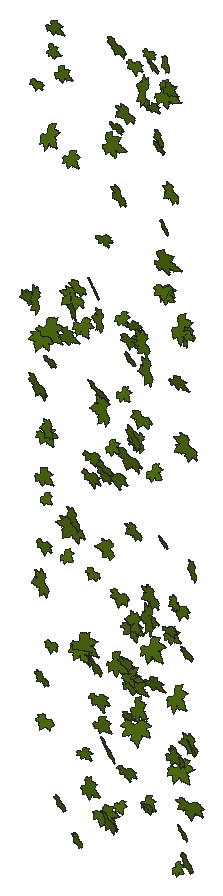
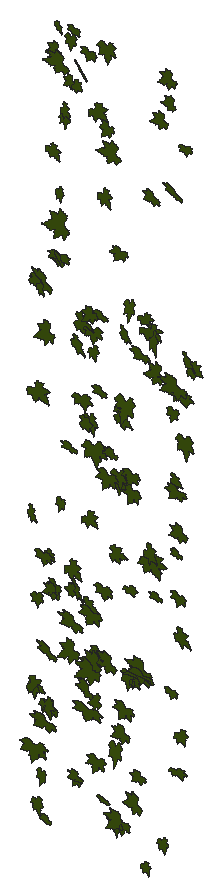
# SketchUp Ruby script. Lengths in inches.
U = 1.inch
M = Sketchup.active_model
def pt(a) = Geom::Point3d.new(a.map { |v| v * U })
def face(e, loops, mat)
  f = e.add_face(loops[0].map { |a| pt(a) })
  loops[1..].each { |l| e.add_face(l.map { |a| pt(a) }).erase! }
  f.material = f.back_material = mat if mat
  f
end
# faces: each face lists its corners as indices into pts; further lists are holes
def faces(e, pts, list, mat = nil) = list.each { |f| face(e, (f[0].is_a?(Array) ? f : [f]).map { |l| l.map { |i| pts[i] } }, mat) }
# xy, xz, yz: faces in a plane at the given z, y or x. An outline is a flat list of corners, or four numbers for a rectangle; further outlines are holes
def ring(l) = l.size == 4 ? [[l[0], l[1]], [l[2], l[1]], [l[2], l[3]], [l[0], l[3]]] : l.each_slice(2).to_a
def flat(e, list, mat, &to3) = list.each { |f| face(e, (f[0].is_a?(Array) ? f : [f]).map { |l| ring(l).map { |u, v| to3.(u, v) } }, mat) }
def xy(e, z, list, mat = nil) = flat(e, list, mat) { |x, y| [x, y, z] }
def xz(e, y, list, mat = nil) = flat(e, list, mat) { |x, z| [x, y, z] }
def yz(e, x, list, mat = nil) = flat(e, list, mat) { |y, z| [x, y, z] }
def lines(e, pts, list) = list.each { |a, b| e.add_line(pt(pts[a]), pt(pts[b])) }
# prism: a flat outline (further loops are holes) pulled along v
def prism(e, loops, v, mat = nil)
  f = face(e, loops, mat); d = Geom::Vector3d.new(v.map { |x| x * U })
  f.pushpull(f.normal.samedirection?(d) ? d.length : -d.length)
end
def box(e, o, s, mat = nil) = prism(e, [[o, [o[0] + s[0], o[1], o[2]], [o[0] + s[0], o[1] + s[1], o[2]], [o[0], o[1] + s[1], o[2]]]], [0, 0, s[2]], mat)
def at(x, y, z, deg = 0) = Geom::Transformation.translation(pt([x, y, z])) * Geom::Transformation.rotation(ORIGIN, Z_AXIS, deg.degrees)
def axes(o, x, y, z) = Geom::Transformation.new([*x, 0, *y, 0, *z, 0, *pt(o).to_a, 1])
def part(name) = M.definitions.add(name)
# library, detail: a bought-in or finely detailed component or shape, given as its bounding box
def library(name, o, s) = part(name).tap { |d| box(d.entities, o, s) }
def detail(e, o, s) = box(e.add_group.entities, o, s)
def put(e, d, t, mat = nil) = e.add_instance(d, t).tap { |i| i.material = mat if mat }
def group(e, t, mat = nil) = e.add_group.tap { |g| g.transformation = t; g.material = mat if mat }.entities
root = M.entities
M.materials.add("[Vegetation Blur 03]").color = [83, 114, 18]
c1 = part("ivy")
xy(c1.entities,0,[[0.782,0,0.786,0,0.787,0.005,0.789,0.009,0.821,0.072,0.875,0.147,1.001,0.272,1.073,0.331,1.137,0.363,1.178,0.379,1.223,0.384,1.272,0.383,1.311,0.374,1.36,0.355,1.399,0.334,1.491,0.285,1.541,0.244,1.583,0.199,1.617,0.15,1.64,0.128,1.662,0.115,1.717,0.105,1.745,0.093,1.784,0.054,1.819,0.057,1.854,0.064,1.882,0.075,1.896,0.074,1.91,0.071,1.937,0.063,1.964,0.053,1.99,0.038,2.016,0.015,2.034,0.002,2.04,0,2.038,0.003,2.036,0.007,2.033,0.038,2.036,0.068,2.045,0.1,2.055,0.116,2.064,0.123,2.077,0.129,2.088,0.129,2.106,0.132,2.118,0.13,2.179,0.132,2.207,0.133,2.225,0.133,2.242,0.138,2.22,0.162,2.207,0.186,2.206,0.213,2.212,0.236,2.228,0.262,2.247,0.274,2.298,0.283,2.355,0.294,2.37,0.296,2.376,0.295,2.377,0.3,2.377,0.303,2.385,0.329,2.411,0.37,2.426,0.392,2.449,0.407,2.511,0.426,2.561,0.444,2.619,0.466,2.589,0.469,2.561,0.476,2.501,0.5,2.449,0.516,2.424,0.523,2.401,0.535,2.377,0.556,2.372,0.568,2.36,0.575,2.268,0.586,2.225,0.592,2.207,0.599,2.194,0.61,2.143,0.65,2.13,0.664,2.122,0.682,2.123,0.7,2.13,0.719,2.148,0.75,2.17,0.781,2.195,0.807,2.221,0.828,2.284,0.874,2.291,0.88,2.288,0.887,2.276,0.9,2.267,0.916,2.265,0.933,2.273,0.967,2.292,1.002,2.313,1.03,2.334,1.054,2.348,1.067,2.358,1.074,2.363,1.076,2.362,1.081,2.35,1.094,2.347,1.11,2.35,1.143,2.359,1.18,2.385,1.254,2.415,1.324,2.448,1.393,2.45,1.4,2.446,1.398,2.44,1.394,2.427,1.383,2.402,1.36,2.376,1.339,2.345,1.324,2.305,1.309,2.282,1.303,2.273,1.306,2.245,1.294,2.212,1.287,2.187,1.291,2.163,1.301,2.142,1.316,2.134,1.327,2.124,1.325,2.09,1.292,2.053,1.259,2.014,1.234,1.973,1.215,1.954,1.21,1.931,1.208,1.909,1.212,1.893,1.22,1.879,1.233,1.872,1.248,1.867,1.281,1.864,1.319,1.821,1.258,1.773,1.197,1.726,1.141,1.698,1.121,1.679,1.116,1.666,1.117,1.647,1.122,1.632,1.129,1.62,1.141,1.617,1.154,1.617,1.219,1.621,1.254,1.623,1.268,1.623,1.281,1.618,1.314,1.606,1.346,1.603,1.375,1.607,1.403,1.603,1.467,1.599,1.499,1.605,1.525,1.614,1.552,1.629,1.577,1.635,1.589,1.629,1.587,1.618,1.582,1.596,1.566,1.581,1.556,1.568,1.552,1.557,1.55,1.545,1.553,1.531,1.562,1.522,1.572,1.504,1.591,1.486,1.611,1.474,1.631,1.457,1.666,1.455,1.684,1.457,1.698,1.452,1.715,1.444,1.728,1.424,1.754,1.419,1.772,1.423,1.786,1.434,1.819,1.444,1.848,1.446,1.855,1.44,1.861,1.43,1.867,1.386,1.904,1.349,1.948,1.326,1.973,1.31,1.995,1.288,2.048,1.284,2.153,1.287,2.254,1.284,2.255,1.282,2.253,1.278,2.247,1.274,2.237,1.266,2.216,1.226,2.125,1.208,2.076,1.184,2.033,1.155,1.984,1.135,1.942,1.111,1.899,1.083,1.861,1.053,1.85,1.059,1.83,1.061,1.809,1.056,1.79,1.049,1.767,1.04,1.749,1.018,1.733,0.994,1.726,0.942,1.734,0.95,1.6875,0.944,1.645,0.932,1.608,0.911,1.585,0.881,1.58,0.854,1.582,0.828,1.588,0.785,1.618,0.773,1.625,0.775,1.614,0.779,1.598,0.796,1.502,0.818,1.402,0.861,1.283,0.882,1.224,0.894,1.174,0.892,1.148,0.886,1.123,0.881,1.107,0.872,1.099,0.849,1.094,0.818,1.092,0.789,1.098,0.762,1.107,0.753,1.113,0.721,1.139,0.698,1.163,0.678,1.194,0.665,1.224,0.628,1.28,0.612,1.312,0.606,1.327,0.606,1.314,0.599,1.282,0.594,1.267,0.581,1.256,0.544,1.245,0.512,1.244,0.473,1.249,0.444,1.256,0.382,1.288,0.339,1.306,0.324,1.316,0.317,1.324,0.309,1.326,0.27,1.314,0.227,1.313,0.185,1.3125,0.152,1.317,0.122,1.328,0.092,1.345,0.073,1.353,0.079,1.338,0.092,1.308,0.117,1.249,0.13,1.215,0.139,1.164,0.147,1.148,0.157,1.136,0.163,1.122,0.174,1.086,0.177,1.067,0.182,1.054,0.186,1.043,0.191,1.038,0.211,1.028,0.237,1.005,0.25,0.974,0.253,0.96,0.25,0.944,0.242,0.914,0.243,0.906,0.249,0.902,0.26,0.894,0.289,0.88,0.307,0.873,0.322,0.862,0.364,0.799,0.403,0.738,0.431,0.709,0.439,0.691,0.441,0.678,0.4375,0.66,0.428,0.645,0.394,0.623,0.303,0.594,0.255,0.581,0.214,0.577,0.179,0.573,0.173,0.568,0.175,0.561,0.167,0.55,0.141,0.523,0.113,0.503,0.077,0.49,0.045,0.486,0.026,0.485,0.019,0.486,0.011,0.483,0,0.471,0.014,0.467,0.044,0.455,0.058,0.447,0.07,0.438,0.097,0.411,0.125,0.394,0.158,0.377,0.174,0.366,0.182,0.359,0.185,0.361,0.242,0.331,0.253,0.316,0.258,0.303,0.262,0.283,0.274,0.278,0.308,0.274,0.341,0.252,0.366,0.226,0.366,0.222,0.37,0.22,0.38,0.221,0.395,0.221,0.425,0.216,0.45,0.207,0.465,0.192,0.473,0.178,0.484,0.15,0.489,0.116,0.483,0.089,0.468,0.058,0.45,0.035,0.435,0.018,0.429,0.011,0.434,0.012,0.438,0.014,0.469,0.019,0.542,0.016,0.581,0.015,0.612,0.027,0.68,0.055,0.696,0.057,0.712,0.052,0.73,0.045,0.741,0.036,0.766,0.014]])
put(root,c1,axes([10.54,173.2,129.93],[0.13601,0.05917,-0.30855],[-0.37908,0.03752,-0.11017],[-0.00748,-0.82593,-0.02711]),"[Vegetation Blur 03]")
put(root,c1,axes([11.16,173.2,130.28],[0.14174,-0.20689,-0.42841],[-0.51411,0.25268,-0.13249],[-0.14609,-1.08996,0.0506]),"[Vegetation Blur 03]")
put(root,c1,axes([10.64,173.2,141.22],[0.29737,0.00668,-0.03254],[-0.03987,-0.00069,-0.24271],[0.00326,-0.6174,-0.00008]),"[Vegetation Blur 03]")
put(root,c1,axes([10.58,173.2,125.73],[0.57169,-0.21875,-0.18427],[-0.21197,0.1873,-0.473],[-0.13171,-1.2509,-0.0386]),"[Vegetation Blur 03]")
put(root,c1,axes([11.09,173.2,110.08],[0.26898,-0.00531,-0.22272],[-0.27011,0.10743,-0.21769],[-0.03898,-0.78115,-0.02842]),"[Vegetation Blur 03]")
put(root,c1,axes([11.41,173.2,115.51],[0.26861,-0.16753,-0.42435],[-0.51691,0.14174,-0.22674],[-0.09889,-1.19591,0.03257]),"[Vegetation Blur 03]")
put(root,c1,axes([10.76,173.2,128.02],[0.48108,0.0091,-0.09014],[-0.10924,-0.11608,-0.39016],[0.0169,-1.00907,0.04407]),"[Vegetation Blur 03]")
put(root,c1,axes([11.17,173.2,107.875],[0.36198,-0.00364,-0.10329],[-0.12566,-0.10485,-0.29275],[0.01516,-0.7821,0.03972]),"[Vegetation Blur 03]")
put(root,c1,axes([10.77,173.2,120.11],[0.22933,0.01454,0.32661],[0.40022,0.004,-0.18721],[0.0052,-0.94915,0.00421]),"[Vegetation Blur 03]")
put(root,c1,axes([10.95,173.2,117.01],[0.4011,-0.07198,0.04538],[0.05521,-0.01426,-0.32859],[-0.0356,-0.83315,0.0017]),"[Vegetation Blur 03]")
put(root,c1,axes([11.83,173.2,123.52],[0.12968,-0.11784,-0.31424],[-0.38451,0.09135,-0.11108],[-0.06065,-0.83104,0.03235]),"[Vegetation Blur 03]")
put(root,c1,axes([11.125,173.2,119.08],[0.14273,0.06127,0.20808],[0.25666,-0.04237,-0.11531],[-0.00355,-0.59977,0.0294]),"[Vegetation Blur 03]")
put(root,c1,axes([10.82,173.2,122.49],[0.3729,0.07352,0.23123],[0.28448,-0.01242,-0.30497],[0.02479,-0.96364,0.02157]),"[Vegetation Blur 03]")
put(root,c1,axes([11.37,173.2,126.86],[0.33145,-0.08577,-0.02014],[-0.01771,0.11215,-0.26935],[-0.04508,-0.6747,-0.04221]),"[Vegetation Blur 03]")
put(root,c1,axes([10.73,173.2,127.82],[0.38163,0.10723,0.44815],[0.5511,-0.01709,-0.31195],[0.0229,-1.37595,0.0388]),"[Vegetation Blur 03]")
put(root,c1,axes([11.05,173.2,138.07],[0.21319,0.1755,0.40106],[0.49372,-0.23014,-0.15897],[-0.07069,-1.078,0.09923]),"[Vegetation Blur 03]")
put(root,c1,axes([11.49,173.2,111.84],[0.32221,-0.0387,0.02273],[0.02664,-0.04287,-0.26295],[-0.0205,-0.66413,0.01565]),"[Vegetation Blur 03]")
put(root,c1,axes([11.57,173.2,142.77],[0.07701,-0.01607,0.28736],[0.35217,-0.0014,-0.06288],[-0.00233,-0.74167,-0.00611]),"[Vegetation Blur 03]")
put(root,c1,axes([11.4375,173.2,144.13],[0.23882,-0.04134,0.29544],[0.36225,0.06442,-0.19363],[0.01513,-0.89011,-0.02773]),"[Vegetation Blur 03]")
put(root,c1,axes([12.13,173.2,103.89],[0.29522,-0.08617,-0.18688],[-0.21829,0.16177,-0.24143],[-0.08083,-0.75161,-0.03054]),"[Vegetation Blur 03]")
put(root,c1,axes([11.95,173.2,141.74],[0.16739,0.00231,0.3142],[0.38437,0.04772,-0.13645],[0.02172,-0.86254,-0.00671]),"[Vegetation Blur 03]")
put(root,c1,axes([12.29,173.2,116.37],[0.12441,0.10653,0.22366],[0.27873,-0.02631,-0.1013],[0.00957,-0.61876,0.04281]),"[Vegetation Blur 03]")
put(root,c1,axes([12.51,173.2,118.875],[0.56655,-0.0115,-0.27779],[-0.34007,0.04247,-0.46224],[-0.01542,-1.35941,-0.01209]),"[Vegetation Blur 03]")
put(root,c1,axes([12.84,173.2,130.89],[0.41729,-0.27977,-0.39423],[-0.44817,0.37379,-0.3577],[-0.22574,-1.25924,-0.01859]),"[Vegetation Blur 03]")
put(root,c1,axes([13.2,173.2,119.35],[0.21226,-0.08156,-0.39258],[-0.47103,0.20087,-0.17619],[-0.10528,-1.06312,-0.00317]),"[Vegetation Blur 03]")
put(root,c1,axes([12.26,173.2,127.98],[0.16066,-0.07376,0.37357],[0.45903,0.04715,-0.13002],[0.00982,-0.99714,-0.03378]),"[Vegetation Blur 03]")
put(root,c1,axes([12.93,173.2,131.1],[0.38856,-0.00058,-0.29483],[-0.35992,-0.09405,-0.31593],[0.03091,-1.0877,0.02748]),"[Vegetation Blur 03]")
put(root,c1,axes([12.41,173.2,137.5],[0.24024,0.06291,0.29442],[0.3619,-0.06648,-0.19446],[-0.01006,-0.88941,0.03536]),"[Vegetation Blur 03]")
put(root,c1,axes([13.27,173.2,102.25],[0.22842,-0.06235,-0.19773],[-0.23665,0.11144,-0.18763],[-0.06007,-0.67607,-0.01269]),"[Vegetation Blur 03]")
put(root,c1,axes([13.18,173.2,131.52],[0.31144,-0.00755,-0.1936],[-0.23722,0.00118,-0.25419],[-0.00327,-0.80561,0.00144]),"[Vegetation Blur 03]")
put(root,c1,axes([12.76,173.2,111.87],[0.43423,0.11965,0.28912],[0.35873,-0.10053,-0.35232],[0.01383,-1.14881,0.06094]),"[Vegetation Blur 03]")
put(root,c1,axes([12.99,173.2,128.98],[0.34318,0.09184,0.26358],[0.326,-0.10859,-0.27677],[-0.00403,-0.96364,0.05631]),"[Vegetation Blur 03]")
put(root,c1,axes([13.25,173.2,106.47],[0.24944,0.02336,0.19362],[0.23616,0.05082,-0.20362],[0.02524,-0.70655,-0.00824]),"[Vegetation Blur 03]")
put(root,c1,axes([13.93,173.2,111.9],[0.17883,0.01791,-0.19414],[-0.23754,0.05276,-0.14498],[-0.01529,-0.61012,-0.01823]),"[Vegetation Blur 03]")
put(root,c1,axes([12.83,173.2,111.91],[0.34678,0.03788,0.46084],[0.56412,0.05104,-0.28341],[0.03077,-1.36263,0.00219]),"[Vegetation Blur 03]")
put(root,c1,axes([13.64,173.2,122.55],[0.40772,-0.01716,0.08723],[0.10718,0.04684,-0.33224],[-0.00228,-0.8661,-0.01969]),"[Vegetation Blur 03]")
put(root,c1,axes([14.08,173.2,116.62],[0.28445,-0.01133,-0.1134],[-0.139,-0.04223,-0.23156],[0.00407,-0.65007,0.01702]),"[Vegetation Blur 03]")
put(root,c1,axes([14.01,173.2,131.88],[0.40706,-0.21039,-0.21028],[-0.21941,0.3311,-0.33502],[-0.1694,-0.93442,-0.07136]),"[Vegetation Blur 03]")
put(root,c1,axes([13.52,173.2,104.53],[0.18345,-0.01602,0.41607],[0.50825,-0.08298,-0.14976],[-0.04057,-1.11184,0.00518]),"[Vegetation Blur 03]")
put(root,c1,axes([13.6,173.2,121.625],[0.48848,-0.12647,0.08295],[0.10536,0.05262,-0.40062],[-0.05484,-1.02537,-0.03079]),"[Vegetation Blur 03]")
put(root,c1,axes([14.01,173.2,111.94],[0.464,-0.18688,-0.09777],[-0.10719,0.14954,-0.38378],[-0.10541,-0.97473,-0.04013]),"[Vegetation Blur 03]")
put(root,c1,axes([14.87,173.2,130.38],[0.12813,-0.15006,-0.36786],[-0.44192,0.20151,-0.11546],[-0.11482,-0.94298,0.03387]),"[Vegetation Blur 03]")
put(root,c1,axes([13.9375,173.2,126.54],[0.61753,-0.18671,-0.12394],[-0.12621,0.33022,-0.49708],[-0.12397,-1.26626,-0.11135]),"[Vegetation Blur 03]")
put(root,c1,axes([15.15,173.2,125.98],[0.21628,-0.19716,-0.4852],[-0.59473,0.13393,-0.18514],[-0.09444,-1.29492,0.05473]),"[Vegetation Blur 03]")
put(root,c1,axes([13.97,173.2,109.84],[0.46672,-0.03992,0.15461],[0.18977,0.01161,-0.3811],[-0.01585,-1.03645,-0.01022]),"[Vegetation Blur 03]")
put(root,c1,axes([14.35,173.2,134.17],[0.33638,0.01493,0.11781],[0.14294,0.07701,-0.27338],[0.02139,-0.74929,-0.02575]),"[Vegetation Blur 03]")
put(root,c1,axes([14.21,173.2,108.24],[0.25126,-0.00237,0.3092],[0.37875,0.02524,-0.20497],[0.00958,-0.93516,-0.00632]),"[Vegetation Blur 03]")
put(root,c1,axes([14.5625,173.2,122.54],[0.44154,-0.10792,-0.13293],[-0.15664,0.11844,-0.36167],[-0.06888,-0.96117,-0.02964]),"[Vegetation Blur 03]")
put(root,c1,axes([14.58,173.2,122.13],[0.39751,-0.09835,-0.09675],[-0.112,0.11608,-0.32505],[-0.0616,-0.84567,-0.03337]),"[Vegetation Blur 03]")
put(root,c1,axes([15.46,173.2,118.44],[0.06394,-0.03491,-0.38067],[-0.46672,-0.01334,-0.05203],[0.00412,-0.96871,0.01444]),"[Vegetation Blur 03]")
put(root,c1,axes([14.11,173.2,103.51],[0.43162,0.02667,0.37239],[0.45622,0.01814,-0.35241],[0.01531,-1.29236,0.00274]),"[Vegetation Blur 03]")
put(root,c1,axes([14.76,173.2,107.9],[0.51252,-0.27009,-0.18144],[-0.18784,0.30748,-0.42542],[-0.17711,-1.10772,-0.07385]),"[Vegetation Blur 03]")
put(root,c1,axes([14.82,173.2,104.04],[0.4822,-0.17189,-0.16775],[-0.19534,0.15084,-0.39833],[-0.10519,-1.06807,-0.02926]),"[Vegetation Blur 03]")
put(root,c1,axes([14.97,173.2,123.02],[0.11399,0.08931,0.26369],[0.32563,0.00233,-0.09389],[0.01551,-0.70503,0.03309]),"[Vegetation Blur 03]")
put(root,c1,axes([14.81,173.2,138.76],[0.09049,0.02962,0.47011],[0.57571,0.04471,-0.07426],[0.0237,-1.19903,0.00884]),"[Vegetation Blur 03]")
put(root,c1,axes([15.18,173.2,145.125],[0.51011,-0.11701,-0.13612],[-0.15838,0.15628,-0.41647],[-0.07724,-1.09327,-0.04497]),"[Vegetation Blur 03]")
put(root,c1,axes([15.6875,173.2,137.34],[0.31562,-0.0779,-0.30416],[-0.3657,0.1532,-0.25894],[-0.08116,-0.99323,-0.01608]),"[Vegetation Blur 03]")
put(root,c1,axes([14.9375,173.2,122.03],[0.51598,-0.04836,0.08245],[0.10256,0.07999,-0.4201],[-0.01553,-1.07898,-0.03484]),"[Vegetation Blur 03]")
put(root,c1,axes([15.17,173.2,140.5],[0.35213,-0.1038,0.09821],[0.12718,0.11373,-0.28482],[-0.02917,-0.75727,-0.05624]),"[Vegetation Blur 03]")
put(root,c1,axes([15.01,173.2,111.54],[0.19537,0.05525,0.44525],[0.54604,-0.05051,-0.1586],[-0.01409,-1.19141,0.02737]),"[Vegetation Blur 03]")
put(root,c1,axes([15.39,173.2,115.97],[0.45876,-0.06676,-0.02085],[-0.02631,-0.02088,-0.37522],[-0.03182,-0.94526,0.00976]),"[Vegetation Blur 03]")
put(root,c1,axes([15.49,173.2,104.47],[0.21181,0.06558,0.16158],[0.19963,-0.12494,-0.16633],[-0.01894,-0.58339,0.05378]),"[Vegetation Blur 03]")
put(root,c1,axes([16.14,173.2,141.78],[0.26725,0.04128,-0.32232],[-0.39537,0.00799,-0.21819],[0.00802,-0.98126,-0.01534]),"[Vegetation Blur 03]")
put(root,c1,axes([15.53,173.2,130.23],[0.21448,0.07418,0.20841],[0.25788,-0.06923,-0.1729],[-0.00284,-0.68276,0.04017]),"[Vegetation Blur 03]")
put(root,c1,axes([15.59,173.2,126.15],[0.18344,0.08958,0.24161],[0.29922,-0.05038,-0.14838],[0.0019,-0.7149,0.04073]),"[Vegetation Blur 03]")
put(root,c1,axes([15.67,173.2,106.68],[0.44484,-0.01751,0.04002],[0.04967,0.10203,-0.36079],[-0.00297,-0.91526,-0.04099]),"[Vegetation Blur 03]")
put(root,c1,axes([15.73,173.2,112.36],[0.36338,-0.06137,0.0857],[0.10665,0.03955,-0.29676],[-0.02326,-0.77736,-0.02186]),"[Vegetation Blur 03]")
put(root,c1,axes([15.78,173.2,123.66],[0.62172,-0.07982,-0.18766],[-0.22411,0.16779,-0.50577],[-0.06444,-1.35373,-0.05162]),"[Vegetation Blur 03]")
put(root,c1,axes([16.27,173.2,128.71],[0.25042,-0.03463,-0.18206],[-0.21423,0.16131,-0.2011],[-0.06442,-0.671,-0.03895]),"[Vegetation Blur 03]")
put(root,c1,axes([15.95,173.2,129.65],[0.43667,-0.00599,-0.05285],[-0.0643,0.07555,-0.35518],[-0.00825,-0.90526,-0.02929]),"[Vegetation Blur 03]")
put(root,c1,axes([16.05,173.2,109.36],[0.12453,-0.12682,0.21988],[0.27637,0.0612,-0.0987],[0.00185,-0.60769,-0.05583]),"[Vegetation Blur 03]")
put(root,c1,axes([16.62,173.2,119.83],[0.24891,0.01709,-0.28911],[-0.35411,0.04401,-0.20266],[-0.01273,-0.88984,-0.01558]),"[Vegetation Blur 03]")
put(root,c1,axes([17.07,173.2,115.13],[0.07751,-0.08641,-0.39879],[-0.48715,0.10409,-0.06661],[-0.05668,-1.01274,0.02718]),"[Vegetation Blur 03]")
put(root,c1,axes([16.42,173.2,124.97],[0.45681,-0.21004,-0.23078],[-0.27305,0.15298,-0.3819],[-0.12578,-1.09491,-0.00909]),"[Vegetation Blur 03]")
put(root,c1,axes([15.99,173.2,111.1875],[0.0827,0.01826,0.45445],[0.55686,-0.01784,-0.06738],[-0.00727,-1.15829,0.0082]),"[Vegetation Blur 03]")
put(root,c1,axes([15.875,173.2,114.28],[0.50405,-0.0121,0.1413],[0.17315,0.00073,-0.4114],[-0.00545,-1.09673,-0.00183]),"[Vegetation Blur 03]")
put(root,c1,axes([16.11,173.2,130.17],[0.30561,-0.04373,0.17256],[0.21196,0.11676,-0.24539],[0.01507,-0.75575,-0.0479]),"[Vegetation Blur 03]")
put(root,c1,axes([16.27,173.2,144.17],[0.38022,-0.03036,0.06928],[0.08439,-0.02832,-0.31043],[-0.01739,-0.80118,0.00835]),"[Vegetation Blur 03]")
put(root,c1,axes([17.29,173.2,124.72],[0.06632,-0.08264,-0.34848],[-0.42857,0.02082,-0.0551],[-0.0162,-0.88896,0.0311]),"[Vegetation Blur 03]")
put(root,c1,axes([15.89,173.2,110.95],[0.37722,-0.01424,0.37521],[0.45787,0.12358,-0.30587],[0.04206,-1.2175,-0.03543]),"[Vegetation Blur 03]")
put(root,c1,axes([15.92,173.2,109.12],[0.61342,0.08443,0.16311],[0.20359,-0.16924,-0.49623],[0.01316,-1.31678,0.07424]),"[Vegetation Blur 03]")
put(root,c1,axes([17.44,173.2,130.22],[0.15478,-0.07462,-0.45486],[-0.55676,0.07347,-0.12809],[-0.04416,-1.18802,0.02065]),"[Vegetation Blur 03]")
put(root,c1,axes([16.7,173.2,125.87],[0.44969,-0.01244,-0.10758],[-0.13185,-0.00591,-0.36702],[-0.00499,-0.96429,0.00364]),"[Vegetation Blur 03]")
put(root,c1,axes([17.65,173.2,143.54],[0.07293,-0.28065,-0.423],[-0.50755,0.30955,-0.09059],[-0.17213,-1.03162,0.0879]),"[Vegetation Blur 03]")
put(root,c1,axes([16.44,173.2,109.63],[0.13579,0.06981,0.42324],[0.51409,-0.17958,-0.1052],[-0.07611,-1.08841,0.0445]),"[Vegetation Blur 03]")
put(root,c1,axes([17.52,173.2,142.51],[0.10604,0.023,-0.23018],[-0.28135,0.05824,-0.08542],[-0.02259,-0.61729,-0.01663]),"[Vegetation Blur 03]")
put(root,c1,axes([17.62,173.2,128.93],[0.29092,-0.24551,-0.40873],[-0.49509,0.19114,-0.25278],[-0.14116,-1.1764,0.04423]),"[Vegetation Blur 03]")
put(root,c1,axes([17.78,173.2,115.91],[0.26701,-0.30376,-0.4486],[-0.53833,0.27065,-0.24226],[-0.1847,-1.22801,0.05757]),"[Vegetation Blur 03]")
put(root,c1,axes([17.67,173.2,116.89],[0.30205,-0.06223,-0.36549],[-0.44449,0.11303,-0.2477],[-0.06243,-1.1058,-0.00475]),"[Vegetation Blur 03]")
put(root,c1,axes([17.1,173.2,105.14],[0.28399,-0.06546,0.07539],[0.09562,0.06624,-0.23087],[-0.02006,-0.61097,-0.03311]),"[Vegetation Blur 03]")
put(root,c1,axes([17.03,173.2,105.02],[0.18546,0.05213,0.26962],[0.33131,-0.03649,-0.15069],[-0.00311,-0.77875,0.02511]),"[Vegetation Blur 03]")
put(root,c1,axes([17.26,173.2,145.09],[0.3174,-0.05029,0.04385],[0.05287,-0.02687,-0.25971],[-0.02626,-0.66189,0.00721]),"[Vegetation Blur 03]")
put(root,c1,axes([17.49,173.2,144.76],[0.35771,-0.12648,-0.10441],[-0.11497,0.1604,-0.29291],[-0.08323,-0.76513,-0.04414]),"[Vegetation Blur 03]")
put(root,c1,axes([17.35,173.2,122.53],[0.15249,0.14355,0.27563],[0.34484,-0.05498,-0.12257],[0.00385,-0.76056,0.06089]),"[Vegetation Blur 03]")
put(root,c1,axes([16.93,173.2,113.11],[0.33086,0.13392,0.42114],[0.51995,-0.11554,-0.26631],[-0.01255,-1.25609,0.0694]),"[Vegetation Blur 03]")
put(root,c1,axes([17.45,173.2,142.08],[0.20167,-0.04503,0.17751],[0.21848,0.0617,-0.16287],[0.00725,-0.60725,-0.02971]),"[Vegetation Blur 03]")
put(root,c1,axes([17.59,173.2,114.78],[0.04043,-0.04833,0.23762],[0.29161,-0.02839,-0.03396],[-0.01694,-0.60422,-0.01741]),"[Vegetation Blur 03]")
put(root,c1,axes([18.18,173.2,141.07],[0.17412,-0.05091,-0.27988],[-0.33267,0.17495,-0.14285],[-0.08689,-0.77186,-0.01392]),"[Vegetation Blur 03]")
put(root,c1,axes([17.22,173.2,111.6],[0.33482,-0.12296,0.29954],[0.37174,0.13576,-0.26801],[0.00918,-1.01326,-0.07226]),"[Vegetation Blur 03]")
put(root,c1,axes([17.88,173.2,140.47],[0.29211,-0.05666,-0.12031],[-0.1385,0.15286,-0.23529],[-0.05752,-0.65573,-0.04445]),"[Vegetation Blur 03]")
put(root,c1,axes([18.36,173.2,136.44],[0.23798,-0.09799,-0.20106],[-0.2294,0.19812,-0.19604],[-0.10166,-0.67644,-0.02829]),"[Vegetation Blur 03]")
put(root,c1,axes([18.13,173.2,119.7],[0.31001,-0.14403,-0.03677],[-0.03088,0.13304,-0.25536],[-0.0773,-0.63077,-0.04546]),"[Vegetation Blur 03]")
put(root,c1,axes([17.85,173.2,132.83],[0.4392,0.07424,0.06802],[0.08567,-0.05755,-0.35857],[0.03015,-0.91812,0.02798]),"[Vegetation Blur 03]")
put(root,c1,axes([18.61,173.2,145.22],[0.22954,-0.17233,-0.19599],[-0.23774,0.09106,-0.19805],[-0.09034,-0.67751,0.02323]),"[Vegetation Blur 03]")
put(root,c1,axes([17.87,173.2,142.5],[0.13182,0.09274,0.49871],[0.61259,0.00582,-0.10802],[0.01227,-1.28635,0.03547]),"[Vegetation Blur 03]")
put(root,c1,axes([18.16,173.2,132.14],[0.09631,0.08819,0.32844],[0.40359,-0.08421,-0.07527],[-0.03009,-0.84734,0.04167]),"[Vegetation Blur 03]")
put(root,c1,axes([17.88,173.2,133.74],[0.17934,-0.09894,0.51265],[0.6295,0.08025,-0.14425],[0.02442,-1.34184,-0.04643]),"[Vegetation Blur 03]")
put(root,c1,axes([18.8,173.2,138.62],[0.34594,-0.11487,-0.25725],[-0.31497,0.04827,-0.28551],[-0.05712,-0.96184,0.01639]),"[Vegetation Blur 03]")
put(root,c1,axes([18.33,173.2,114.89],[0.3213,-0.06644,0.14929],[0.18483,0.03966,-0.26218],[-0.01845,-0.75978,-0.02674]),"[Vegetation Blur 03]")
put(root,c1,axes([18.33,173.2,143.24],[0.18668,-0.06069,0.28857],[0.35478,0.02187,-0.15215],[-0.00434,-0.8225,-0.02534]),"[Vegetation Blur 03]")
put(root,c1,axes([18.4,173.2,114.36],[0.19136,0.01715,0.31471],[0.38568,-0.01715,-0.15606],[-0.00376,-0.88569,0.00911]),"[Vegetation Blur 03]")
put(root,c1,axes([19.1,173.2,116.86],[0.2154,-0.10325,-0.19292],[-0.23671,0.04089,-0.17948],[-0.04859,-0.65681,0.01915]),"[Vegetation Blur 03]")
put(root,c1,axes([18.97,173.2,108.93],[0.42245,-0.13873,-0.23601],[-0.28027,0.15555,-0.34853],[-0.09809,-1.04193,-0.02061]),"[Vegetation Blur 03]")
put(root,c1,axes([18.53,173.2,108.1],[0.22931,-0.05412,0.29769],[0.36487,-0.02596,-0.18795],[-0.02469,-0.88622,-0.01267]),"[Vegetation Blur 03]")
put(root,c1,axes([18.93,173.2,102.15],[0.08845,0.08211,0.23234],[0.28731,-0.04554,-0.07032],[-0.00952,-0.61175,0.03642]),"[Vegetation Blur 03]")
put(root,c1,axes([18.54,173.2,110.93],[0.19869,0.16598,0.44202],[0.5434,-0.20587,-0.15053],[-0.06748,-1.16914,0.08926]),"[Vegetation Blur 03]")
put(root,c1,axes([18.52,173.2,107.34],[0.3778,0.16016,0.36511],[0.45377,-0.08873,-0.30663],[0.01685,-1.20168,0.0713]),"[Vegetation Blur 03]")
put(root,c1,axes([19.7,173.2,131.13],[0.17466,-0.11177,-0.29584],[-0.34642,0.21964,-0.14928],[-0.11976,-0.79834,0.00035]),"[Vegetation Blur 03]")
put(root,c1,axes([18.71,173.2,128],[0.29936,-0.14494,0.31849],[0.3965,0.0953,-0.24142],[-0.00556,-1.00761,-0.06865]),"[Vegetation Blur 03]")
put(root,c1,axes([18.98,173.2,116.53],[0.44619,-0.06474,-0.00167],[-0.00306,-0.02944,-0.36486],[-0.03138,-0.91771,0.01182]),"[Vegetation Blur 03]")
put(root,c1,axes([19.29,173.2,104.83],[0.35108,-0.18402,-0.07774],[-0.07773,0.15757,-0.29247],[-0.10502,-0.7318,-0.04343]),"[Vegetation Blur 03]")
put(root,c1,axes([19.67,173.2,125.68],[0.41789,-0.06408,-0.38347],[-0.47,0.02266,-0.34176],[-0.02893,-1.29377,0.01301]),"[Vegetation Blur 03]")
put(root,c1,axes([18.82,173.2,130.47],[0.16468,0.13945,0.51477],[0.63081,-0.17776,-0.12684],[-0.06707,-1.32961,0.07095]),"[Vegetation Blur 03]")
put(root,c1,axes([19.62,173.2,103.47],[0.35757,-0.14861,-0.22341],[-0.2596,0.18993,-0.29662],[-0.11295,-0.907,-0.02551]),"[Vegetation Blur 03]")
put(root,c1,axes([19.52,173.2,114.33],[0.32932,-0.07979,-0.11263],[-0.13041,0.12861,-0.26832],[-0.05951,-0.72344,-0.03528]),"[Vegetation Blur 03]")
put(root,c1,axes([20.21,173.2,109.84],[0.13243,-0.0083,-0.40164],[-0.49158,0.04791,-0.10811],[-0.02353,-1.04762,-0.00176]),"[Vegetation Blur 03]")
put(root,c1,axes([20.12,173.2,131.3125],[0.07838,0.01913,-0.25028],[-0.30675,-0.00782,-0.06408],[0.00599,-0.6513,-0.00658]),"[Vegetation Blur 03]")
put(root,c1,axes([20.26,173.2,118.95],[0.13696,-0.09293,-0.32969],[-0.38837,0.22901,-0.11762],[-0.11998,-0.84735,0.00437]),"[Vegetation Blur 03]")
put(root,c1,axes([19.79,173.2,109.54],[0.33215,-0.12492,-0.16924],[-0.19211,0.18741,-0.2729],[-0.09889,-0.78367,-0.03828]),"[Vegetation Blur 03]")
put(root,c1,axes([19.18,173.2,106.25],[0.6157,0.01002,0.02515],[0.03061,0.04996,-0.50212],[0.00607,-1.26758,-0.01959]),"[Vegetation Blur 03]")
